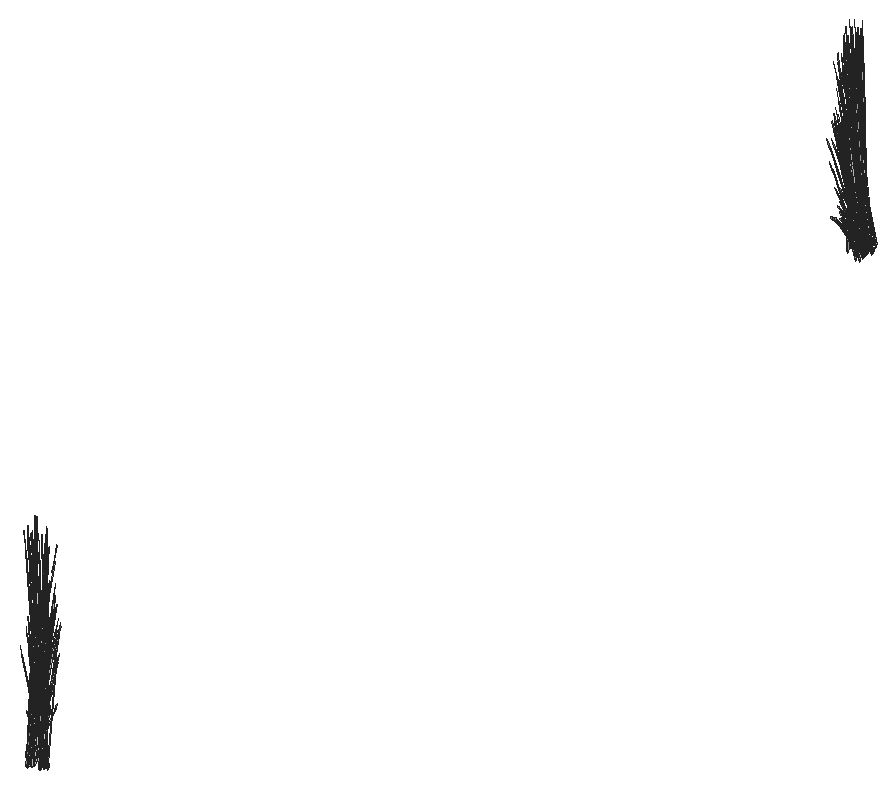
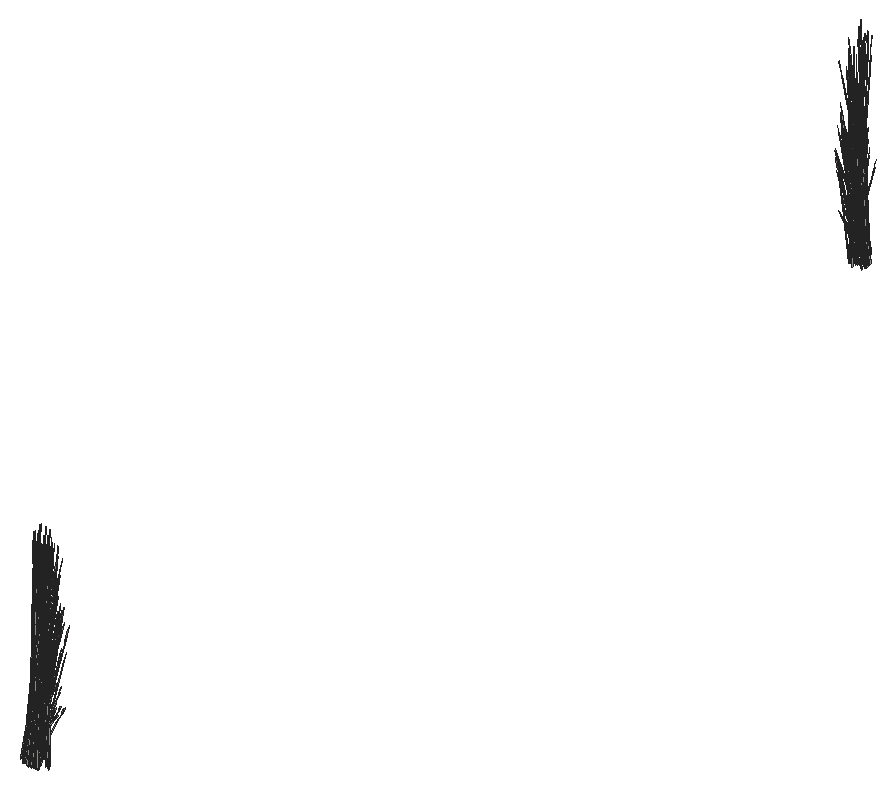
# SketchUp Ruby script. Lengths in inches.
U = 1.inch
M = Sketchup.active_model
def pt(a) = Geom::Point3d.new(a.map { |v| v * U })
def face(e, loops, mat)
  f = e.add_face(loops[0].map { |a| pt(a) })
  loops[1..].each { |l| e.add_face(l.map { |a| pt(a) }).erase! }
  f.material = f.back_material = mat if mat
  f
end
# faces: each face lists its corners as indices into pts; further lists are holes
def faces(e, pts, list, mat = nil) = list.each { |f| face(e, (f[0].is_a?(Array) ? f : [f]).map { |l| l.map { |i| pts[i] } }, mat) }
# xy, xz, yz: faces in a plane at the given z, y or x. An outline is a flat list of corners, or four numbers for a rectangle; further outlines are holes
def ring(l) = l.size == 4 ? [[l[0], l[1]], [l[2], l[1]], [l[2], l[3]], [l[0], l[3]]] : l.each_slice(2).to_a
def flat(e, list, mat, &to3) = list.each { |f| face(e, (f[0].is_a?(Array) ? f : [f]).map { |l| ring(l).map { |u, v| to3.(u, v) } }, mat) }
def xy(e, z, list, mat = nil) = flat(e, list, mat) { |x, y| [x, y, z] }
def xz(e, y, list, mat = nil) = flat(e, list, mat) { |x, z| [x, y, z] }
def yz(e, x, list, mat = nil) = flat(e, list, mat) { |y, z| [x, y, z] }
def lines(e, pts, list) = list.each { |a, b| e.add_line(pt(pts[a]), pt(pts[b])) }
# prism: a flat outline (further loops are holes) pulled along v
def prism(e, loops, v, mat = nil)
  f = face(e, loops, mat); d = Geom::Vector3d.new(v.map { |x| x * U })
  f.pushpull(f.normal.samedirection?(d) ? d.length : -d.length)
end
def box(e, o, s, mat = nil) = prism(e, [[o, [o[0] + s[0], o[1], o[2]], [o[0] + s[0], o[1] + s[1], o[2]], [o[0], o[1] + s[1], o[2]]]], [0, 0, s[2]], mat)
def at(x, y, z, deg = 0) = Geom::Transformation.translation(pt([x, y, z])) * Geom::Transformation.rotation(ORIGIN, Z_AXIS, deg.degrees)
def axes(o, x, y, z) = Geom::Transformation.new([*x, 0, *y, 0, *z, 0, *pt(o).to_a, 1])
def part(name) = M.definitions.add(name)
# library, detail: a bought-in or finely detailed component or shape, given as its bounding box
def library(name, o, s) = part(name).tap { |d| box(d.entities, o, s) }
def detail(e, o, s) = box(e.add_group.entities, o, s)
def put(e, d, t, mat = nil) = e.add_instance(d, t).tap { |i| i.material = mat if mat }
def group(e, t, mat = nil) = e.add_group.tap { |g| g.transformation = t; g.material = mat if mat }.entities
root = M.entities
M.materials.add("LightPink_Translucent").color = [144, 107, 117]
M.materials["LightPink_Translucent"].alpha = 0.75
c1 = part("blade")
p = [[2.15,0.21,22],[0,0.17,0],[0.09,0.45,0],[2.18,0.31,22],[2.29,0.31,22],[0.38,0.45,0],
  [2.48,0.24,33],[2.49,0.24,33],[2.48,0.22,33]]
faces(c1.entities,p,[[0,1,2,3],[4,5,2,3],[6,3,4,7],[8,0,3,6]])
c2 = part("seeds")
p = [[0.3,-0.1,1.38],[-0.01,-0.03,1.59],[-0.01,-0.03,0.03],[0.14,-0.07,-0.07],[0.29,-0.03,3],[0.15,0.01,3.11]]
faces(c2.entities,p,[[0,1,2,3],[1,0,4,5]],"LightPink_Translucent")
c3 = part("blade with seeds")
put(c3.entities,c1,at(0,0,0))
put(c3.entities,c2,axes([2.4,0.25,30.99],[1.5799,-0.05474,1.17369],[-0.12525,1.92788,0.29478],[-0.07173,-0.02425,1.56792]))
put(root,c3,axes([338.03,356.94,623.05],[0.1064,-0.35863,0.35414],[0.31043,0.1046,-0.4572],[0.02846,0.14439,0.87481]))
put(root,c3,axes([336.875,649.7,622.1],[0.22066,-0.46731,0],[0.36918,0.26061,-0.51607],[0.08408,0.05936,1.63711]))
put(root,c3,axes([337.24,649.49,621.22],[-0.05283,-0.03674,1.76342],[-0.13569,-0.41045,-0.26939],[0.09154,-0.11138,0.30037]))
put(root,c3,axes([341.11,649.42,624.42],[0.02617,0.04654,1.77383],[-0.12614,0.41836,-0.16761],[-0.12775,0.00303,0.31391]))
put(root,c3,axes([338.61,356.35,620.29],[0.15345,0.53576,-0.06012],[-0.43845,0.18773,0],[0.00536,0.01871,1.72173]))
put(root,c3,axes([340.05,651.92,621.66],[0.09355,-0.55261,-0.23429],[0.44354,0.09633,0.51271],[-0.0775,-0.07631,1.5644]))
put(root,c3,axes([341.4,649.15,624.42],[-0.07594,-0.00329,1.74944],[-0.24177,0.32918,-0.27667],[-0.129,-0.06726,0.14031]))
put(root,c3,axes([340.63,355.97,622.68],[0.09067,0.42583,-0.51099],[-0.34336,0.07449,-0.3958],[-0.0984,0.11438,0.97773]))
put(root,c3,axes([340.09,356.74,622.72],[-0.00877,0.09229,1.74944],[0.24897,0.32105,-0.27667],[-0.06518,0.15182,0.14031]))
put(root,c3,axes([337.23,650.48,624.4],[-0.09067,-0.42583,-0.51099],[0.34336,-0.07449,-0.3958],[0.0984,-0.11438,0.97773]))
put(root,c3,axes([340.17,648.43,623.9375],[-0.05398,-0.06539,1.74944],[-0.36026,0.04145,-0.27667],[-0.0575,-0.15639,0.14031]))
put(root,c3,axes([338.1,357,622.98],[0.16845,0.3792,-0.71045],[-0.34676,0.21133,0.08574],[0.03939,0.18322,1.00501]))
put(root,c3,axes([339.875,355.64,620.2],[-0.44111,-0.00373,-0.04976],[0,-0.52122,0.49943],[-0.01386,0.11865,1.58352]))
put(root,c3,axes([340.0625,649.5,621.44],[-0.10181,0.3808,-0.03893],[-0.31336,-0.11714,-0.17649],[-0.04758,-0.06228,0.58215]))
put(root,c3,axes([338.91,650.89,621.24],[0,-0.46636,-0.49651],[0.39487,0,0],[0,-0.10622,1.57504]))
put(root,c3,axes([339.08,651.32,621.7],[0,0.46636,0.49651],[-0.39487,0,0],[0,-0.10622,1.57504]))
put(root,c3,axes([341.6,649.97,624.74],[-0.0189,0.47427,-0.1216],[-0.35781,-0.01296,-0.67495],[-0.13781,-0.03295,1.02557]))
put(root,c3,axes([341.375,650,624.23],[-0.20082,-0.29199,-0.35414],[0.2293,-0.2764,0.4572],[-0.1165,-0.04206,0.87481]))
put(root,c3,axes([342.33,355.35,621.875],[0.12246,-0.09864,1.71376],[0.1031,0.45582,0.13857],[-0.19225,0.10302,0.73262]))
put(root,c3,axes([340.88,648.21,624.03],[-0.00658,0.0559,1.77383],[-0.32474,0.20287,-0.16761],[-0.09556,-0.1037,0.31391]))
put(root,c3,axes([340.53,649.02,621.91],[-0.02137,0.15256,1.43002],[-0.31245,0.12771,-0.30754],[-0.07303,-0.19719,0.61141]))
put(root,c3,axes([341.95,356.125,620.59],[0.12266,0.03828,1.43002],[0.07906,0.39104,-0.30754],[-0.16661,0.0732,0.61141]))
put(root,c3,axes([338.45,358.22,623.65],[0.2439,-0.26754,-0.06488],[0.22348,0.29302,-0.29416],[0.01573,0.08303,0.97024]))
put(root,c3,axes([340.63,649.42,623.19],[0.08068,0.14973,1.71376],[-0.3728,0.12606,0.13857],[-0.08426,-0.23506,0.73262]))
put(root,c3,axes([340.89,650.7,622.47],[0.22533,-0.03337,1.1486],[-0.14293,0.29403,0.84392],[-0.11135,-0.04411,0.25299]))
put(root,c3,axes([339.95,651.43,621.89],[-0.39748,-0.22252,-0.29095],[0.19139,-0.46966,-0.50002],[-0.01249,-0.11531,1.59708]))
put(root,c3,axes([338.88,355.0625,620.72],[0.17124,-0.42022,0.44739],[0.35581,0.20224,-0.21531],[0,0.09687,1.43643]))
put(root,c3,axes([338.73,356.52,620.2],[0.35581,0.20937,0],[-0.17124,0.43505,0],[0,0,1.74954]))
put(root,c3,axes([337.66,649.63,622.49],[-0.11756,0.2374,1.1486],[-0.10105,-0.31895,0.84392],[0.09709,-0.07992,0.25299]))
put(root,c3,axes([340.47,355.67,623.03],[0.32648,0.25715,-0.1216],[-0.18809,0.3724,-0.67495],[-0.09224,0.12945,1.02557]))
put(root,c3,axes([340.76,649.34,623.84],[-0.05451,-0.37564,-0.35414],[0.31161,-0.09919,0.4572],[-0.0837,-0.10765,0.87481]))
put(root,c3,axes([337.52,650.6875,624.45],[0.2423,0.19613,0.0643],[-0.14107,0.2793,0.50621],[0.07768,-0.0903,0.77189]))
put(root,c3,axes([343.04,354.87,621.34],[0.10032,-0.06746,1.77064],[0.0346,0.47103,0.13857],[-0.2173,0.0625,0.63284]))
put(root,c3,axes([339.89,651.24,621.69],[-0.44133,0,0],[0,-0.52122,-0.51607],[0,-0.11871,1.63711]))
put(root,c3,axes([338.23,357.08,622.68],[0.34695,0.11691,-0.51099],[-0.11892,0.40083,-0.3958],[0.03181,0.16138,0.97773]))
put(root,c3,axes([337.93,357.1,623.03],[0.34538,-0.21713,-0.1216],[0.16972,0.38536,-0.67495],[0.04557,0.16239,1.02557]))
put(root,c3,axes([341.21,356.84,620.375],[-0.22066,0.46731,0],[-0.36918,-0.26061,-0.51607],[-0.08408,-0.05936,1.63711]))
put(root,c3,axes([337.45,650.61,624.46],[0.08753,0.42921,0.48003],[-0.34336,0.07449,0.3958],[0.1012,-0.10094,0.9933]))
put(root,c3,axes([341.34,649.89,624.8],[0.29147,-0.34417,0.53763],[0.25138,0.3655,0.4433],[-0.13675,-0.06349,1.11249]))
put(root,c3,axes([339.77,650.95,621.32],[-0.14494,-0.47823,-0.69835],[0.41752,-0.17223,-0.18329],[-0.01602,-0.16194,1.54149]))
put(root,c3,axes([340.72,649.43,624.26],[-0.34538,0.21713,-0.1216],[-0.16972,-0.38536,-0.67495],[-0.04557,-0.16239,1.02557]))
put(root,c3,axes([340.42,649.45,623.9],[-0.34695,-0.11691,-0.51099],[0.11892,-0.40083,-0.3958],[-0.03181,-0.16138,0.97773]))
put(root,c3,axes([339.78,355.72,620.03],[-0.24637,0.29097,-0.30978],[-0.24637,-0.29097,0.30978],[0,0.09372,1.38974]))
put(root,c3,axes([339.93,356.79,623.65],[0.31145,0.12449,-0.06488],[-0.0958,0.38314,-0.29416],[-0.05094,0.05817,0.97024]))
put(root,c3,axes([340.95,649.65,624.37],[0.05451,0.37564,0.35414],[-0.31161,0.09919,-0.4572],[-0.0837,-0.10765,0.87481]))
put(root,c3,axes([339.08,355.67,620.09],[0.12941,0.42699,-0.69212],[-0.37279,0.15378,-0.18165],[0.0143,0.14459,1.52773]))
put(root,c3,axes([341.96,355.1875,622.72],[-0.05763,0.06055,1.74944],[0.0049,0.44239,-0.27667],[-0.13211,0.05753,0.14031]))
put(root,c3,axes([340.23,651.1,621.65],[-0.32829,0.39208,0.30756],[-0.32849,-0.38796,-0.36492],[-0.01146,-0.11134,1.64885]))
put(root,c3,axes([338.2,650.67,624.43],[-0.0461,-0.00354,1.77383],[-0.19143,-0.37951,-0.16761],[0.07688,-0.12478,0.31391]))
put(root,c3,axes([339.08,650.9,621.25],[0.24637,-0.29097,-0.30978],[0.24637,0.29097,0.30978],[0,-0.09372,1.38974]))
put(root,c3,axes([340.63,355.7,623.05],[0.30722,-0.06665,0.35414],[0.08112,0.381,-0.4572],[-0.08804,0.10234,0.87481]))
put(root,c3,axes([343.08,650.62,623.6],[0.14639,-0.01056,1.71376],[-0.09712,0.45778,0.13857],[-0.20862,-0.02831,0.73262]))
put(root,c3,axes([340.19,649.02,621.35],[-0.2439,0.26754,-0.03893],[-0.22348,-0.29302,-0.17649],[-0.01573,-0.08303,0.58215]))
put(root,c3,axes([339.03,355.16,620.62],[0.32884,-0.136,0.1448],[0.11516,0.38837,-0.41347],[0,0.08547,1.26744]))
put(root,c3,axes([340.8,357.52,620.59],[0.11138,-0.07357,1.43002],[0.27499,0.22183,-0.30754],[-0.08185,0.19194,0.61141]))
put(root,c3,axes([341.59,652.1875,622.64],[0.305,0.18805,1.51261],[-0.29879,0.40513,0.59816],[-0.13384,-0.24012,1.26806]))
put(root,c3,axes([337.49,650.52,624.25],[0.30722,-0.06665,-0.35414],[0.08112,0.381,0.4572],[0.08804,-0.10234,0.87481]))
put(root,c3,axes([337.24,650.65,624.71],[0.18436,-0.36797,-0.71045],[0.32306,0.26151,0.08574],[0.11008,-0.13332,1.00501]))
put(root,c3,axes([340.42,648.78,622.08],[0.18411,0.16231,1.1486],[-0.26813,0.09757,0.84392],[-0.05737,-0.12474,0.25299]))
put(root,c3,axes([341.09,651.7,621.53],[-0.21202,-0.39143,-0.44739],[0.32115,-0.27564,0.21531],[-0.06861,-0.04843,1.43643]))
put(root,c3,axes([337.41,651.79,624.76],[-0.17758,-0.42229,-0.1216],[0.31518,-0.20752,-0.67495],[0.13282,-0.05572,1.02557]))
put(root,c3,axes([340.55,649.53,624.21],[-0.16845,-0.3792,-0.71045],[0.34676,-0.21133,0.08574],[-0.03939,-0.18322,1.00501]))
put(root,c3,axes([338.92,355.19,620.67],[0.39748,0.22252,-0.29095],[-0.19139,0.46966,-0.50002],[0.01249,0.11531,1.59708]))
put(root,c3,axes([341.48,649.89,624.4375],[0.01777,-0.35463,0.0643],[0.26836,0.00972,0.50621],[-0.1028,-0.03711,0.77189]))
put(root,c3,axes([340.81,649.2,624.41],[0.39316,-0.11987,0.53763],[0.06823,0.47021,0.4433],[-0.09247,-0.13858,1.11249]))
put(root,c3,axes([341.32,355.63,622.71],[0.04504,0.01251,1.77383],[0.13934,0.41205,-0.16761],[-0.0922,0.10815,0.31391]))
put(root,c3,axes([342.3,649.27,625.14],[-0.23555,0.44708,-0.13619],[-0.34112,-0.25757,-0.75594],[-0.11858,-0.12631,1.14864]))
put(root,c3,axes([342.34,355.13,622.68],[-0.09562,0.42421,-0.51099],[-0.32782,-0.1454,-0.3958],[-0.13199,0.0389,0.97773]))
put(root,c3,axes([340.92,356.72,622.73],[-0.25132,-0.3182,0.48003],[0.2669,-0.27442,0.3958],[-0.04636,0.14929,0.9933]))
put(root,c3,axes([341.66,650.15,624.76],[0.20082,0.29199,0.35414],[-0.2293,0.2764,-0.4572],[-0.1165,-0.04206,0.87481]))
put(root,c3,axes([342.2,649.64,624.6875],[-0.30095,-0.22541,-0.71045],[0.21388,-0.395,0.08574],[-0.10904,-0.13459,1.00501]))
put(root,c3,axes([340.9,649.3,624.05],[0.16041,-0.29625,0.0643],[0.22843,0.17248,0.50621],[-0.07385,-0.09498,0.77189]))
put(root,c3,axes([342.06,649.65,624.39],[-0.34827,0.11086,-0.51099],[-0.06092,-0.41983,-0.3958],[-0.09354,-0.12031,0.97773]))
put(root,c3,axes([340.83,356.69,622.73],[-0.29004,-0.02173,0.0643],[0.00795,-0.32812,0.50621],[-0.03035,0.12569,0.77189]))
put(root,c3,axes([339.78,355.3,620.48],[0,-0.46636,0.49651],[0.39487,0,0],[0,0.10622,1.57504]))
put(root,c3,axes([339.95,355.73,620.02],[0,0.46636,-0.49651],[-0.39487,0,0],[0,0.10622,1.57504]))
put(root,c3,axes([338.9,357.14,622.73],[-0.35104,0.10702,0.48003],[-0.06092,-0.41983,0.3958],[0.08256,0.12373,0.9933]))
put(root,c3,axes([340.61,649.59,624.28],[-0.1064,0.35863,0.35414],[-0.31043,-0.1046,-0.4572],[-0.02846,-0.14439,0.87481]))
put(root,c3,axes([338.83,357.22,622.73],[-0.16041,0.29625,0.0643],[-0.22843,-0.17248,0.50621],[0.07385,0.09498,0.77189]))
put(root,c3,axes([340.92,356.8125,622.53],[-0.23881,0.24554,-0.35414],[-0.22606,-0.28036,0.4572],[-0.0344,0.14245,0.87481]))
put(root,c3,axes([338.42,356.25,621.875],[-0.08068,-0.14973,1.71376],[0.3728,-0.12606,0.13857],[0.08426,0.23506,0.73262]))
put(root,c3,axes([341.125,651.92,621.76],[0.09355,-0.55261,-0.23429],[0.44354,0.09633,0.51271],[-0.0775,-0.07631,1.5644]))
put(root,c3,axes([341.61,649.27,621.2],[-0.03419,0.06144,1.76342],[-0.3455,0.13246,-0.26939],[-0.08346,-0.12049,0.30037]))
put(root,c3,axes([337.39,651.42,624.4],[0.09562,-0.42421,-0.51099],[0.32782,0.1454,-0.3958],[0.13199,-0.0389,0.97773]))
put(root,c3,axes([341.69,356.94,620.77],[0.14709,-0.21136,1.1486],[0.05804,0.3346,0.84392],[-0.1063,0.05991,0.25299]))
put(root,c3,axes([342.14,356.08,620.06],[-0.23773,0.35053,-0.62353],[-0.29532,-0.31785,-0.16365],[-0.09526,0.08744,1.37633]))
put(root,c3,axes([340.07,357.68,622.71],[0.04004,-0.02816,1.77383],[0.33095,0.18728,-0.16761],[-0.00778,0.15594,0.31391]))
put(root,c3,axes([341.25,648.43,624.03],[-0.05398,-0.06539,1.74944],[-0.36026,0.04145,-0.27667],[-0.0575,-0.15639,0.14031]))
put(root,c3,axes([339.99,650.89,621.33],[0,-0.46636,-0.49651],[0.39487,0,0],[0,-0.10622,1.57504]))
put(root,c3,axes([340.16,651.32,621.8],[0,0.46636,0.49651],[-0.39487,0,0],[0,-0.10622,1.57504]))
put(root,c3,axes([337.51,650.3125,622.31],[-0.12609,-0.01381,1.43002],[-0.12917,-0.37055,-0.30754],[0.1549,-0.10482,0.61141]))
put(root,c3,axes([342.33,354.77,623.03],[0.17758,0.42229,-0.1216],[-0.31518,0.20752,-0.67495],[-0.13282,0.05572,1.02557]))
put(root,c3,axes([342.3,355.88,620.46],[-0.34464,-0.37536,-0.25192],[0.29,-0.42149,0.5513],[-0.0928,0.04391,1.68216]))
put(root,c3,axes([342.78,355.65,621.875],[0.08815,-0.14329,1.71376],[0.22258,0.38678,0.13857],[-0.15267,0.17614,0.73262]))
put(root,c3,axes([342.25,356.03,622.53],[-0.30722,0.06665,-0.35414],[-0.08112,-0.381,0.4572],[-0.08804,0.10234,0.87481]))
put(root,c3,axes([340.26,648.6875,620.72],[-0.0592,0.0168,1.76342],[-0.32738,-0.18913,-0.26939],[0.00549,-0.15776,0.30037]))
put(root,c3,axes([341.08,356.55,623.34],[-0.00918,0.43138,-0.7886],[-0.38672,-0.02897,0.09517],[-0.04081,0.18275,1.11556]))
put(root,c3,axes([341.02,651.43,621.98],[-0.39748,-0.22252,-0.29095],[0.19139,-0.46966,-0.50002],[-0.01249,-0.11531,1.59708]))
put(root,c3,axes([342.08,357.16,619.49],[0.04734,0.04659,1.76342],[0.08027,0.4317,-0.26939],[-0.10492,0.09206,0.30037]))
put(root,c3,axes([340.58,649.21,623.75],[0.1064,-0.35863,-0.35414],[0.31043,0.1046,0.4572],[-0.02846,-0.14439,0.87481]))
put(root,c3,axes([338.78,356.88,623.05],[-0.05451,-0.37564,0.35414],[0.31161,-0.09919,-0.4572],[0.0837,0.10765,0.87481]))
put(root,c3,axes([340.06,651.14,621.58],[0.15345,0.52148,0.45755],[-0.43845,0.18134,0.17955],[0.00536,-0.09582,1.58856]))
put(root,c3,axes([341.07,357.76,620.77],[-0.00913,-0.2773,1.1486],[0.22824,0.19778,0.84392],[-0.04489,0.13217,0.25299]))
put(root,c3,axes([339.99,651.08,621.43],[0.17124,-0.42022,-0.44739],[0.35581,0.20224,0.21531],[0,-0.09687,1.43643]))
put(root,c3,axes([343.52,650.19,624.71],[-0.35281,-0.01123,-0.71045],[0.0237,-0.47284,0.08574],[-0.14947,-0.0499,1.00501]))
put(root,c3,axes([341.4,649.5,621.84],[-0.10181,0.3808,-0.03893],[-0.31336,-0.11714,-0.17649],[-0.04758,-0.06228,0.58215]))
put(root,c3,axes([342.13,355.8,620.21],[-0.38326,0.02879,-0.44739],[-0.03466,-0.47788,0.21531],[-0.06861,0.04843,1.43643]))
put(root,c3,axes([338.85,354.92,620.21],[0.21202,0.39143,-0.44739],[-0.32115,0.27564,0.21531],[0.06861,0.04843,1.43643]))
put(root,c3,axes([343.24,650.31,622.32],[0.06891,0.12984,1.43002],[-0.15879,0.35293,-0.30754],[-0.16304,-0.08436,0.61141]))
put(root,c3,axes([338.99,354.72,622.47],[-0.30498,-0.24231,1.38283],[0.32203,-0.37727,0.59665],[0.0984,0.22736,1.33663]))
put(root,c3,axes([342.29,355.95,622.73],[-0.08753,-0.42921,0.48003],[0.34336,-0.07449,0.3958],[-0.1012,0.10094,0.9933]))
put(root,c3,axes([342.21,648.21,624.42],[-0.00658,0.0559,1.77383],[-0.32474,0.20287,-0.16761],[-0.09556,-0.1037,0.31391]))
put(root,c3,axes([343.36,649.89,623.6],[0.1311,0.08035,1.71376],[-0.27131,0.33708,0.13857],[-0.16909,-0.15206,0.73262]))
put(root,c3,axes([340.85,650.95,621.41],[-0.14494,-0.47823,-0.69835],[0.41752,-0.17223,-0.18329],[-0.01602,-0.16194,1.54149]))
put(root,c3,axes([341.79,649.43,624.35],[-0.34538,0.21713,-0.1216],[-0.16972,-0.38536,-0.67495],[-0.04557,-0.16239,1.02557]))
put(root,c3,axes([338.48,357.41,622.71],[0.00104,-0.05646,1.77383],[0.30246,-0.2491,-0.16761],[0.10506,0.08891,0.31391]))
put(root,c3,axes([341.86,649.02,622.3],[-0.02137,0.15256,1.43002],[-0.31245,0.12771,-0.30754],[-0.07303,-0.19719,0.61141]))
put(root,c3,axes([341.5,649.45,624],[-0.34695,-0.11691,-0.51099],[0.11892,-0.40083,-0.3958],[-0.03181,-0.16138,0.97773]))
put(root,c3,axes([339.45,356.7,620.77],[-0.19872,-0.13409,1.1486],[0.2566,-0.13625,0.84392],[0.06921,0.11541,0.25299]))
put(root,c3,axes([341.4,356.6,620.48],[0.33032,0.23318,0.49651],[-0.19744,0.41812,0],[-0.07523,-0.05311,1.57504]))
put(root,c3,axes([338.74,356.55,620.59],[0.00623,-0.15459,1.43002],[0.29764,-0.17268,-0.30754],[0.09188,0.18503,0.61141]))
put(root,c3,axes([341.97,649.42,623.58],[0.08068,0.14973,1.71376],[-0.3728,0.12606,0.13857],[-0.08426,-0.23506,0.73262]))
put(root,c3,axes([340.95,357.16,621.36],[0.00775,-0.24075,1.54345],[0.34877,0.12716,0.21329],[-0.03022,0.25658,0.72882]))
put(root,c3,axes([342.22,355.86,622.73],[-0.2423,-0.19613,0.0643],[0.14107,-0.2793,0.50621],[-0.07768,0.0903,0.77189]))
put(root,c3,axes([342.1,649.34,624.23],[-0.05451,-0.37564,-0.35414],[0.31161,-0.09919,0.4572],[-0.0837,-0.10765,0.87481]))
put(root,c3,axes([340.16,650.9,621.35],[0.24637,-0.29097,-0.30978],[0.24637,0.29097,0.30978],[0,-0.09372,1.38974]))
put(root,c3,axes([341.27,649.02,621.44],[-0.2439,0.26754,-0.03893],[-0.22348,-0.29302,-0.17649],[-0.01573,-0.08303,0.58215]))
put(root,c3,axes([341.23,651.24,622.08],[-0.44133,0,0],[0,-0.52122,-0.51607],[0,-0.11871,1.63711]))
put(root,c3,axes([342.71,356.01,621.875],[0.06572,-0.16029,1.71376],[0.27569,0.33172,0.13857],[-0.12437,0.20675,0.73262]))
put(root,c3,axes([343.4,650.29,624.41],[-0.25628,0.30892,-0.51099],[-0.22444,-0.32634,-0.3958],[-0.13021,-0.047,0.97773]))
put(root,c3,axes([342.53,357.03,620.02],[-0.33032,0.23318,-0.49651],[-0.19744,-0.41812,0],[-0.07523,0.05311,1.57504]))
put(root,c3,axes([340.71,649.26,623.95],[0.26007,-0.1585,0.0643],[0.12729,0.28902,0.50621],[-0.02512,-0.1274,0.77189]))
put(root,c3,axes([338.375,651.125,624.4375],[0.04898,-0.07104,1.74944],[-0.06269,-0.43574,-0.27667],[0.12289,-0.08262,0.14031]))
put(root,c3,axes([342.55,356.91,620.19],[-0.21791,-0.46895,-0.05142],[0.36918,-0.26061,0.51607],[-0.09097,0.04465,1.6363]))
put(root,c3,axes([340.05,355.375,620.375],[0.44133,0,0],[0,0.52122,-0.51607],[0,0.11871,1.63711]))
put(root,c3,axes([340.62,649.29,623.96],[0.34777,0.12192,0.48003],[-0.11892,0.40083,0.3958],[-0.0209,-0.15763,0.9933]))
put(root,c3,axes([340.2,651.29,621.66],[0.39767,0.22603,0.24065],[-0.19139,0.46966,0.50002],[0,-0.10827,1.60543]))
put(root,c3,axes([341.625,649.53,624.3],[-0.16845,-0.3792,-0.71045],[0.34676,-0.21133,0.08574],[-0.03939,-0.18322,1.00501]))
put(root,c3,axes([343.04,649.42,624.43],[0.02617,0.04654,1.77383],[-0.12614,0.41836,-0.16761],[-0.12775,0.00303,0.31391]))
put(root,c3,axes([340.07,650.97,621.94],[-0.38326,0.02879,0.44739],[-0.03466,-0.47788,-0.21531],[0.06861,-0.04843,1.43643]))
put(root,c3,axes([341.16,356.69,623],[0.25266,0.31335,-0.5672],[-0.2669,0.27442,-0.43934],[-0.03844,0.15921,1.08528]))
put(root,c3,axes([342.28,649.65,624.76],[0.05451,0.37564,0.35414],[-0.31161,0.09919,-0.4572],[-0.0837,-0.10765,0.87481]))
put(root,c3,axes([342.5,356.07,622.68],[0.09067,0.42583,-0.51099],[-0.34336,0.07449,-0.3958],[-0.0984,0.11438,0.97773]))
put(root,c3,axes([342.45,356.85,620.03],[-0.32928,-0.11539,-0.30978],[0.08291,-0.40636,0.30978],[-0.06638,0.04686,1.38974]))
put(root,c3,axes([339.48,357.31,620.67],[-0.22633,-0.01463,1.0506],[0.14947,-0.31064,0.58006],[0.08941,0.11036,0.8241]))
put(root,c3,axes([341.04,356.46,623.05],[0.23881,-0.24554,0.35414],[0.22606,0.28036,-0.4572],[-0.0344,0.14245,0.87481]))
put(root,c3,axes([341.57,651.1,622.04],[-0.32829,0.39208,0.30756],[-0.32849,-0.38796,-0.36492],[-0.01146,-0.11134,1.64885]))
put(root,c3,axes([341.97,356.84,622.72],[-0.00877,0.09229,1.74944],[0.24897,0.32105,-0.27667],[-0.06518,0.15182,0.14031]))
put(root,c3,axes([343.33,649.15,624.44],[-0.07594,-0.00329,1.74944],[-0.24177,0.32918,-0.27667],[-0.129,-0.06726,0.14031]))
put(root,c3,axes([342.64,355.11,620.84],[-0.00964,-0.43909,1.41272],[0.43635,0.11382,0.59816],[-0.1032,0.24027,1.3335]))
put(root,c3,axes([342.92,652.1875,623.03],[0.305,0.18805,1.51261],[-0.29879,0.40513,0.59816],[-0.13384,-0.24012,1.26806]))
put(root,c3,axes([341.76,648.78,622.47],[0.18411,0.16231,1.1486],[-0.26813,0.09757,0.84392],[-0.05737,-0.12474,0.25299]))
put(root,c3,axes([343.54,649.97,624.76],[-0.0189,0.47427,-0.1216],[-0.35781,-0.01296,-0.67495],[-0.13781,-0.03295,1.02557]))
put(root,c3,axes([342.43,651.7,621.92],[-0.21202,-0.39143,-0.44739],[0.32115,-0.27564,0.21531],[-0.06861,-0.04843,1.43643]))
put(root,c3,axes([343.31,650,624.25],[-0.20082,-0.29199,-0.35414],[0.2293,-0.2764,0.4572],[-0.1165,-0.04206,0.87481]))
put(root,c3,axes([341.69,649.59,624.37],[-0.1064,0.35863,0.35414],[-0.31043,-0.1046,-0.4572],[-0.02846,-0.14439,0.87481]))
put(root,c3,axes([340.89,356.53,623.4],[0.3879,0.02311,-0.13498],[-0.0106,0.43749,-0.74919],[-0.02694,0.1685,1.13838]))
put(root,c3,axes([339.71,649.58,621.6],[-0.22066,-0.46731,0],[0.36918,-0.26061,-0.51607],[0.08408,-0.05936,1.63711]))
put(root,c3,axes([340.88,357.17,620.82],[0.32063,-0.08258,0.06507],[0.07371,0.33271,-0.86304],[-0.02033,0.16842,0.7736]))
put(root,c3,axes([342.4,355.67,620.67],[0.04113,0.53214,-0.29095],[-0.42835,0.03218,-0.50002],[-0.07543,0.07088,1.59708]))
put(root,c3,axes([338.75,357.08,623.03],[0.21031,-0.39918,-0.1216],[0.30457,0.22997,-0.67495],[0.10587,0.11278,1.02557]))
put(root,c3,axes([342.14,649.2,624.8],[0.39316,-0.11987,0.53763],[0.06823,0.47021,0.4433],[-0.09247,-0.13858,1.11249]))
put(root,c3,axes([341.44,356.25,621.875],[-0.00864,-0.17899,1.71376],[0.37441,0.11874,0.13857],[-0.02316,0.25508,0.73262]))
put(root,c3,axes([344.375,355.26,621.875],[0.12246,-0.09864,1.71376],[0.1031,0.45582,0.13857],[-0.19225,0.10302,0.73262]))
put(root,c3,axes([342.34,355.77,623.03],[0.32648,0.25715,-0.1216],[-0.18809,0.3724,-0.67495],[-0.09224,0.12945,1.02557]))
put(root,c3,axes([342.83,650.7,622.49],[0.22533,-0.03337,1.1486],[-0.14293,0.29403,0.84392],[-0.11135,-0.04411,0.25299]))
put(root,c3,axes([340.63,648.45,621.99],[0.04528,0.27194,1.1486],[-0.25117,-0.15062,0.84392],[0.02703,-0.13924,0.25299]))
put(root,c3,axes([343.08,356.94,620.375],[-0.22066,0.46731,0],[-0.36918,-0.26061,-0.51607],[-0.08408,-0.05936,1.63711]))
put(root,c3,axes([343.99,356.03,620.59],[0.12266,0.03828,1.43002],[0.07906,0.39104,-0.30754],[-0.16661,0.0732,0.61141]))
put(root,c3,axes([342.23,649.3,624.4375],[0.16041,-0.29625,0.0643],[0.22843,0.17248,0.50621],[-0.07385,-0.09498,0.77189]))
put(root,c3,axes([339,356.88,622.68],[0.34827,-0.11086,-0.51099],[0.06092,0.41983,-0.3958],[0.09354,0.12031,0.97773]))
put(root,c3,axes([339.4,356.38,623.05],[-0.20082,-0.29199,0.35414],[0.2293,-0.2764,-0.4572],[0.1165,0.04206,0.87481]))
put(root,c3,axes([343.28,649.89,624.82],[0.29147,-0.34417,0.53763],[0.25138,0.3655,0.4433],[-0.13675,-0.06349,1.11249]))
put(root,c3,axes([341.33,648.6875,620.81],[-0.0592,0.0168,1.76342],[-0.32738,-0.18913,-0.26939],[0.00549,-0.15776,0.30037]))
put(root,c3,axes([342.46,651.92,622.15],[0.09355,-0.55261,-0.23429],[0.44354,0.09633,0.51271],[-0.0775,-0.07631,1.5644]))
put(root,c3,axes([341.8,356.89,623.65],[0.31145,0.12449,-0.06488],[-0.0958,0.38314,-0.29416],[-0.05094,0.05817,0.97024]))
put(root,c3,axes([341.71,648.89,623.93],[-0.03584,0.03562,1.77383],[-0.35118,-0.12018,-0.16761],[-0.01271,-0.15545,0.31391]))
put(root,c3,axes([341.66,649.21,623.84],[0.1064,-0.35863,-0.35414],[0.31043,0.1046,0.4572],[-0.02846,-0.14439,0.87481]))
put(root,c3,axes([339.58,356.64,622.73],[-0.01777,0.35463,0.0643],[-0.26836,-0.00972,0.50621],[0.1028,0.03711,0.77189]))
put(root,c3,axes([341.14,651.14,621.68],[0.15345,0.52148,0.45755],[-0.43845,0.18134,0.17955],[0.00536,-0.09582,1.58856]))
put(root,c3,axes([341.43,649.92,624.26],[-0.3879,-0.02311,-0.1216],[0.0106,-0.43749,-0.67495],[0.02694,-0.1685,1.02557]))
put(root,c3,axes([342.5,355.8,623.05],[0.30722,-0.06665,0.35414],[0.08112,0.381,-0.4572],[-0.08804,0.10234,0.87481]))
put(root,c3,axes([339.51,357.19,619.49],[0.02571,-0.06733,1.76342],[0.32373,-0.19829,-0.26939],[0.09815,0.10263,0.30037]))
put(root,c3,axes([341.07,651.08,621.53],[0.17124,-0.42022,-0.44739],[0.35581,0.20224,0.21531],[0,-0.09687,1.43643]))
put(root,c3,axes([342.58,648.43,624.42],[-0.05398,-0.06539,1.74944],[-0.36026,0.04145,-0.27667],[-0.0575,-0.15639,0.14031]))
put(root,c3,axes([339.61,356.53,622.73],[-0.26024,0.30729,0.48003],[-0.22444,-0.32634,0.3958],[0.1221,0.05668,0.9933]))
put(root,c3,axes([341.33,650.89,621.72],[0,-0.46636,-0.49651],[0.39487,0,0],[0,-0.10622,1.57504]))
put(root,c3,axes([342.68,357.62,620.59],[0.11138,-0.07357,1.43002],[0.27499,0.22183,-0.30754],[-0.08185,0.19194,0.61141]))
put(root,c3,axes([341.5,651.32,622.1875],[0,0.46636,0.49651],[-0.39487,0,0],[0,-0.10622,1.57504]))
put(root,c3,axes([340.28,356.57,621.93],[-0.06755,-0.39203,-0.03492],[0.31928,-0.09013,-0.15832],[0.06667,0.02485,0.52218]))
put(root,c3,axes([341.28,649.99,624.28],[-0.23881,0.24554,0.35414],[-0.22606,-0.28036,-0.4572],[0.0344,-0.14245,0.87481]))
put(root,c3,axes([344,355.1,622.72],[-0.05763,0.06055,1.74944],[0.0049,0.44239,-0.27667],[-0.13211,0.05753,0.14031]))
put(root,c3,axes([342.01,356.4375,620.2],[-0.35581,-0.20937,0],[0.17124,-0.43505,0],[0,0,1.62707]))
put(root,c3,axes([339.04,354.77,620.06],[0.36714,0.07646,-0.62353],[-0.07747,0.47163,-0.16365],[0.10956,0.05715,1.37633]))
put(root,c3,axes([340.14,650.87,621.89],[-0.04113,-0.53214,-0.29095],[0.42835,-0.03218,-0.50002],[0.07543,-0.07088,1.59708]))
put(root,c3,axes([342.83,356.96,620.375],[0.22066,0.46731,0],[-0.36918,0.26061,-0.51607],[-0.08408,0.05936,1.63711]))
